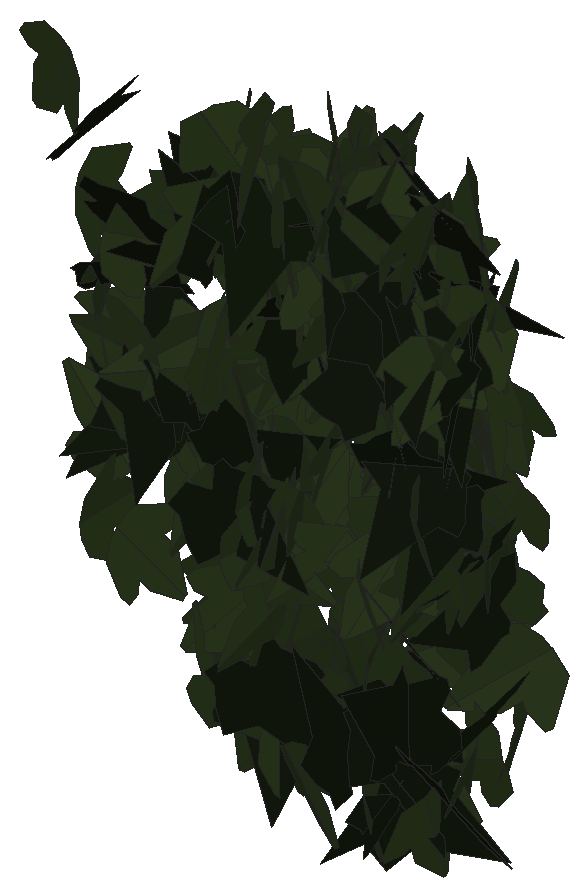
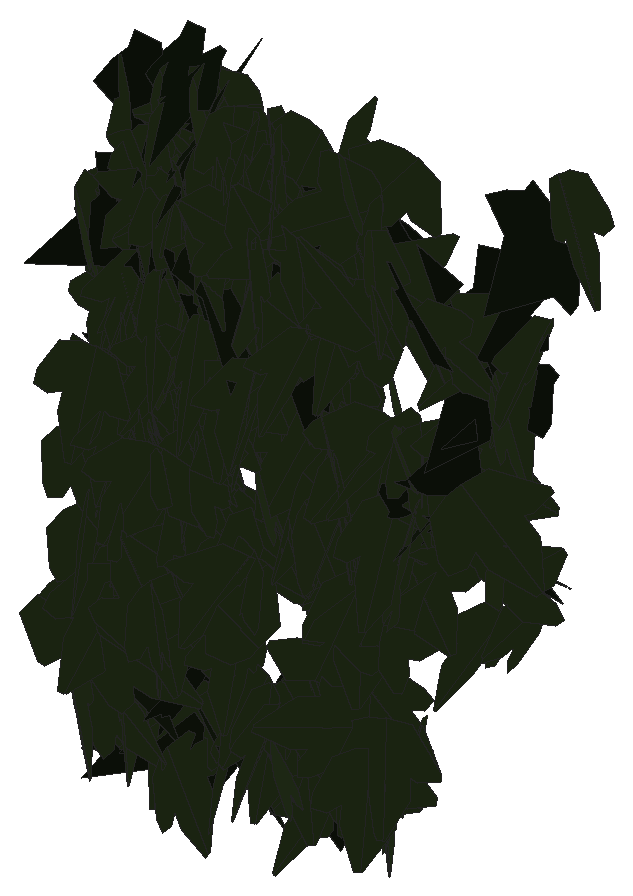
# SketchUp Ruby script. Lengths in inches.
U = 1.inch
M = Sketchup.active_model
def pt(a) = Geom::Point3d.new(a.map { |v| v * U })
def face(e, loops, mat)
  f = e.add_face(loops[0].map { |a| pt(a) })
  loops[1..].each { |l| e.add_face(l.map { |a| pt(a) }).erase! }
  f.material = f.back_material = mat if mat
  f
end
# faces: each face lists its corners as indices into pts; further lists are holes
def faces(e, pts, list, mat = nil) = list.each { |f| face(e, (f[0].is_a?(Array) ? f : [f]).map { |l| l.map { |i| pts[i] } }, mat) }
# xy, xz, yz: faces in a plane at the given z, y or x. An outline is a flat list of corners, or four numbers for a rectangle; further outlines are holes
def ring(l) = l.size == 4 ? [[l[0], l[1]], [l[2], l[1]], [l[2], l[3]], [l[0], l[3]]] : l.each_slice(2).to_a
def flat(e, list, mat, &to3) = list.each { |f| face(e, (f[0].is_a?(Array) ? f : [f]).map { |l| ring(l).map { |u, v| to3.(u, v) } }, mat) }
def xy(e, z, list, mat = nil) = flat(e, list, mat) { |x, y| [x, y, z] }
def xz(e, y, list, mat = nil) = flat(e, list, mat) { |x, z| [x, y, z] }
def yz(e, x, list, mat = nil) = flat(e, list, mat) { |y, z| [x, y, z] }
def lines(e, pts, list) = list.each { |a, b| e.add_line(pt(pts[a]), pt(pts[b])) }
# prism: a flat outline (further loops are holes) pulled along v
def prism(e, loops, v, mat = nil)
  f = face(e, loops, mat); d = Geom::Vector3d.new(v.map { |x| x * U })
  f.pushpull(f.normal.samedirection?(d) ? d.length : -d.length)
end
def box(e, o, s, mat = nil) = prism(e, [[o, [o[0] + s[0], o[1], o[2]], [o[0] + s[0], o[1] + s[1], o[2]], [o[0], o[1] + s[1], o[2]]]], [0, 0, s[2]], mat)
def at(x, y, z, deg = 0) = Geom::Transformation.translation(pt([x, y, z])) * Geom::Transformation.rotation(ORIGIN, Z_AXIS, deg.degrees)
def axes(o, x, y, z) = Geom::Transformation.new([*x, 0, *y, 0, *z, 0, *pt(o).to_a, 1])
def part(name) = M.definitions.add(name)
# library, detail: a bought-in or finely detailed component or shape, given as its bounding box
def library(name, o, s) = part(name).tap { |d| box(d.entities, o, s) }
def detail(e, o, s) = box(e.add_group.entities, o, s)
def put(e, d, t, mat = nil) = e.add_instance(d, t).tap { |i| i.material = mat if mat }
def group(e, t, mat = nil) = e.add_group.tap { |g| g.transformation = t; g.material = mat if mat }.entities
root = M.entities
M.materials.add("efeu1").color = [18, 25, 13]
M.materials.add("efeu2").color = [43, 57, 29]
c1 = part("ivyleaf_10")
p = [[0,0.5,-0.03],[-0.0625,2.02,-0.43],[-0.19,2.01,-0.46],[-0.54,1.05,-0.29],[-0.52,0.625,-0.18],[-0.83,0.76,-0.28],
  [-1.16,0.64,-0.33],[-1.15,0.33,-0.24],[-0.77,-0.39,0.02],[-0.3,-0.51,0.16],[0.04,-0.48,0.23],[-0.02,2.01,-0.4375],
  [-0.06,2.01,-0.43],[0.04,-0.49,0.23],[0.67,-0.49,0.14],[1.38,0.36,-0.2],[1.375,0.51,-0.24],[0.81,0.65,-0.19],
  [0.62,0.59,-0.15],[0.6,1.09,-0.28],[0.5,1.23,-0.31]]
faces(c1.entities,p,[[0,1,2,3,4,5,6,7,8,9,10],[11,12,0,13,14,15,16,17,18,19,20]],"efeu2")
c2 = part("ivyleaf_9")
p = [[1.54,2.16,1.25],[1.36,2.04,1.19],[-0.21,0.99,0.68],[-0.71,1.11,0.82],[-0.85,0.86,0.67],[-0.8,0.17,0.21],
  [-0.9,-0.01,0.1],[-0.67,-0.16,-0.02],[-0.08,-0.08,-0.05],[-0.03,-0.6,-0.4],[0.65,-0.88,-0.66],[0.83,-0.6,-0.49],
  [1.29,-0.42,-0.43],[1.8125,-0.07,-0.26],[1.21,0.44,0.15]]
faces(c2.entities,p,[[0,1,2,3,4,5,6,7,8,9,10,11,12,13,14]],"efeu1")
put(root,c1,axes([5.2,224.04,209.42],[-0.00212,0.02101,0.45187],[-0.16346,0.40731,-0.02119],[-0.44044,-0.15126,0.00569]))
put(root,c2,axes([8.625,224.64,207.9375],[-0.00203,0.05746,0.44843],[-0.23937,-0.37115,0.05043],[0.40424,-0.21948,0.03212]))
put(root,c1,axes([8.18,224.63,208.41],[0.10122,-0.25477,-0.3535],[0.12428,-0.31983,0.28231],[-0.44161,-0.14841,-0.00157]))
put(root,c2,axes([6.96,224.58,213.28],[-0.3714,-0.21956,-0.1569],[0.16606,0.03758,-0.42139],[0.23495,-0.37364,0.04981]))
put(root,c2,axes([8.03,224.45,207.47],[-0.04967,-0.3948,0.18383],[0.04582,0.17278,0.41283],[-0.46492,0.0592,0.02105]))
put(root,c2,axes([8.65,224.39,207.33],[-0.36217,0.27392,-0.04338],[0.03543,-0.02578,-0.45031],[-0.29714,-0.33694,-0.00081]))
put(root,c1,axes([6.83,224.73,208.63],[-0.0006,-0.09982,0.44033],[0.12411,-0.40838,-0.09998],[0.45311,0.11172,0.02797]))
put(root,c1,axes([9.125,224.5,212.34],[0.33338,0.25113,-0.18274],[-0.14436,-0.11411,-0.41383],[-0.29788,0.33636,-0.00396]))
put(root,c2,axes([8.61,224.53,212.71],[-0.21473,-0.29356,-0.2621],[0.19877,0.17748,-0.36601],[0.36755,-0.26748,0.04481]))
put(root,c1,axes([5.54,224.2,209.1875],[0.02158,0.3425,0.27813],[0.0277,0.26632,-0.35671],[-0.46849,0.03152,-0.00828]))
put(root,c1,axes([7.42,224.48,207.21],[-0.31943,0.21184,-0.24801],[0.21615,-0.12999,-0.37824],[-0.26825,-0.357,-0.00945]))
put(root,c2,axes([9,224.62,211.02],[-0.44478,-0.12881,-0.05722],[0.05701,0.01553,-0.44877],[0.14012,-0.4152,0.00096]))
put(root,c2,axes([5.45,224.73,210.68],[-0.06726,-0.41548,0.11732],[-0.00699,-0.11306,-0.4368],[0.46491,-0.06181,0.0104]))
put(root,c2,axes([6.42,224.41,209.95],[-0.03075,-0.08309,-0.44308],[0.34115,0.28887,-0.08054],[0.32153,-0.31444,0.04308]))
put(root,c2,axes([9.26,224.625,210.84],[-0.4243,-0.04481,-0.18856],[0.19735,-0.00503,-0.41051],[0.04165,-0.43266,0.02431]))
put(root,c1,axes([7.2,224.33,209.67],[0.19213,-0.3133,0.25351],[-0.13025,0.21183,0.3747],[-0.40845,-0.21493,-0.00024]))
put(root,c2,axes([8.36,224.52,211.6875],[-0.29043,-0.32348,0.1152],[0.08307,0.08008,0.43741],[-0.35981,0.27959,0.008]))
put(root,c2,axes([4.99,224.41,212.74],[0.41192,-0.06876,0.20544],[0.21519,-0.00554,-0.40211],[0.06873,0.42949,0.0277]))
put(root,c1,axes([8.57,224.42,211.875],[-0.27605,0.34528,0.07114],[-0.05347,0.04843,-0.44663],[-0.37637,-0.26012,0.01127]))
put(root,c1,axes([8.91,224.66,213.81],[0.06813,-0.41929,0.10105],[0.03005,-0.09403,-0.44076],[0.46386,0.06767,0.01371]))
put(root,c1,axes([4.42,224.42,214.15],[0.37791,-0.15784,-0.28682],[-0.19638,0.2412,-0.39148],[0.26194,0.40855,0.12031]))
put(root,c1,axes([9.07,224.31,210.6],[-0.21616,0.22463,0.32675],[-0.23093,0.23023,-0.31286],[-0.34736,-0.29285,0.00466]))
put(root,c1,axes([6.65,224.53,211.17],[-0.27348,0.34702,-0.07117],[0.04419,-0.05486,-0.44677],[-0.37943,-0.2565,-0.00074]))
put(root,c1,axes([9,224.5,207.23],[-0.06491,-0.40687,-0.14734],[0.08934,0.12949,-0.42324],[0.45664,-0.08317,0.06186]))
put(root,c2,axes([6.4,224.38,212.75],[-0.04797,0.10555,0.43644],[-0.2722,0.33661,-0.11579],[-0.37989,-0.25452,0.02785]))
put(root,c1,axes([8.98,224.54,210.05],[-0.41664,0.00882,0.20883],[-0.21705,-0.02308,-0.40051],[0.00307,-0.4343,0.02552]))
put(root,c1,axes([6.11,224.89,212.86],[-0.08756,-0.30933,0.38295],[-0.07097,-0.37696,-0.32072],[0.48713,-0.11052,0.02211]))
put(root,c1,axes([5.1,224.55,209.96],[0.34077,0.14902,0.33417],[-0.33927,-0.04231,0.36484],[0.13702,-0.4754,0.07228]))
put(root,c2,axes([6.86,224.53,208.05],[-0.11147,-0.11457,-0.42302],[0.27588,0.31663,-0.16017],[0.36356,-0.2754,-0.00816]))
put(root,c1,axes([6.62,224.88,213.97],[0.15051,-0.30432,0.36707],[0.22118,-0.29644,-0.33645],[0.4224,0.26366,0.04539]))
put(root,c1,axes([6.81,224.63,209.32],[-0.14118,-0.00993,-0.43137],[0.43765,-0.09638,-0.13042],[-0.09616,-0.42407,0.03974]))
put(root,c2,axes([8.59,224.92,212.67],[-0.07873,-0.39699,0.16868],[-0.02446,-0.16073,-0.41973],[0.46251,-0.07608,0.00651]))
put(root,c1,axes([6.9,224.91,209.53],[0.0196,0.15172,-0.42357],[-0.07247,-0.40177,-0.15876],[-0.46376,0.06919,0.00691]))
put(root,c1,axes([5.33,224.52,211.09],[0.03073,-0.02803,-0.49827],[-0.45328,0.20729,-0.03962],[0.20879,0.45414,-0.01267]))
put(root,c1,axes([7.15,224.62,211.98],[-0.25446,-0.36382,-0.03815],[0.02817,0.02681,-0.45072],[0.39392,-0.23694,0.00759]))
put(root,c1,axes([7.36,224.61,213.74],[-0.42398,0.15176,-0.11432],[0.10621,-0.05035,-0.43756],[-0.17227,-0.40455,0.01157]))
put(root,c2,axes([5.38,224.81,210.63],[-0.46047,-0.08538,0.01283],[-0.01184,-0.00804,-0.45218],[0.09241,-0.42646,0.00596]))
put(root,c1,axes([8.98,224.58,212.38],[-0.44344,0.1425,0.01902],[-0.01907,0.00491,-0.452],[-0.15398,-0.41097,0.0012]))
put(root,c2,axes([4.77,224.28,213.54],[0.15081,0.29111,0.30317],[0.05059,0.29458,-0.32929],[-0.44205,0.13303,0.06574]))
put(root,c1,axes([7.69,224.85,209.49],[-0.16495,-0.19077,0.37426],[-0.23325,-0.28793,-0.25406],[0.37296,-0.26445,0.00663]))
put(root,c1,axes([7,224.6,210.08],[-0.49258,-0.02674,0.08155],[-0.08138,-0.00531,-0.4933],[0.02725,-0.49926,0.00088]))
put(root,c2,axes([8.68,224.44,207.3],[0.02609,-0.03815,-0.44996],[0.14664,0.41226,-0.02992],[0.44556,-0.13345,0.0362]))
put(root,c2,axes([5.13,224.37,212.15],[0.33379,0.28979,0.10256],[0.05012,0.09417,-0.43903],[-0.32678,0.31045,0.03743]))
put(root,c1,axes([8.38,224.44,207.17],[-0.18335,0.31626,0.25556],[-0.15375,0.20181,-0.37241],[-0.40429,-0.22018,0.02573]))
put(root,c1,axes([7.74,224.59,213.72],[0.19435,-0.41858,-0.19242],[-0.05741,0.1852,-0.46087],[0.45709,0.20123,0.02393]))
put(root,c1,axes([8.28,224.51,213.81],[-0.06856,-0.05507,-0.44388],[0.43369,0.14754,-0.08191],[0.16711,-0.40549,0.03048]))
put(root,c1,axes([5.75,224.98,210.94],[-0.01762,0.06632,0.49527],[-0.18417,-0.46155,0.05526],[0.46451,-0.18048,0.0407]))
put(root,c1,axes([8.36,224.75,209.7],[0.38435,0.16569,-0.19491],[-0.18173,-0.08258,-0.40824],[-0.1999,0.39364,-0.00361]))
put(root,c2,axes([8.43,224.7,207.97],[0.13367,-0.43867,-0.19924],[-0.04143,0.19554,-0.45831],[0.48002,0.13903,0.01593]))
put(root,c2,axes([8.47,224.63,210.76],[0.16775,-0.07991,0.41432],[0.42497,-0.07677,-0.17557],[0.10943,0.42065,0.04667]))
put(root,c1,axes([6.89,224.52,212.78],[-0.327,0.1813,0.2645],[-0.24508,0.11569,-0.36673],[-0.23177,-0.37812,0.01461]))
put(root,c2,axes([9.23,224.46,212.06],[-0.29735,0.33575,0.02738],[0.01248,-0.02457,0.45152],[0.36351,0.27548,0.0069]))
put(root,c1,axes([6.23,224.67,213.9],[-0.35741,-0.11571,-0.26783],[0.29682,-0.04122,-0.34804],[0.06978,-0.4173,0.10864]))
put(root,c1,axes([7.09,224.7,213.35],[-0.07337,0.41948,-0.09669],[0.01735,-0.09158,-0.44195],[-0.46371,-0.0698,-0.00123]))
put(root,c1,axes([6.97,224.73,207.53],[-0.36305,-0.16965,0.22652],[-0.21118,-0.09597,-0.3916],[0.2105,-0.38889,-0.00218]))
put(root,c2,axes([8.97,224.7,208.27],[-0.14213,0.01117,-0.43104],[-0.39914,-0.20027,0.11643],[-0.20298,0.386,0.07288]))
put(root,c2,axes([6.46,224.65,210.15],[0.01791,0.00244,0.45206],[0.44631,-0.135,-0.01561],[0.1456,0.41351,-0.00777]))
put(root,c2,axes([8.22,224.66,209.26],[0.43399,-0.16623,-0.01114],[-0.0101,0.00539,-0.45226],[0.17962,0.40195,0.00146]))
put(root,c2,axes([5.53,224.9,210.54],[-0.46135,0.00633,0.08515],[-0.08726,-0.10996,-0.42956],[0.01586,-0.42082,0.11353]))
put(root,c2,axes([8.68,224.72,207.46],[0.40917,-0.18,0.11988],[0.11632,-0.04185,-0.43615],[0.1994,0.39379,0.00844]))
put(root,c1,axes([6.91,224.7,212.68],[-0.46596,-0.00698,-0.05724],[0.05981,-0.02834,-0.44775],[0.00359,-0.43402,0.03016]))
put(root,c2,axes([8.53,225.09,213.37],[0.2317,-0.4172,-0.14919],[0.06983,-0.13187,0.47721],[-0.43754,-0.24198,-0.00285]))
put(root,c1,axes([4.84,224.85,212.12],[0.14378,-0.47608,0.05171],[0.02083,-0.04772,-0.49728],[0.47843,0.14516,0.00611]))
put(root,c2,axes([9.07,224.61,213.89],[0.42077,0.05332,-0.19343],[-0.1997,-0.02051,-0.40894],[-0.06152,0.43123,0.00446]))
put(root,c1,axes([6.72,224.42,209.39],[0.01931,-0.04767,0.44929],[-0.04052,0.43059,0.05103],[-0.46765,-0.03927,0.01413]))
put(root,c1,axes([8.57,224.74,208.58],[-0.37115,-0.03785,0.27455],[-0.28083,-0.04808,-0.35921],[0.06397,-0.43067,0.01597]))
put(root,c1,axes([6.83,224.4375,209.95],[-0.03174,0.02521,0.4506],[-0.21761,0.38384,-0.03744],[-0.41515,-0.20312,-0.01482]))
put(root,c2,axes([9.01,224.88,212.24],[-0.25835,-0.09434,-0.36489],[0.37452,0.06604,-0.26435],[0.11707,-0.41948,0.04045]))
put(root,c2,axes([7.22,224.58,212.11],[0.17541,-0.17371,-0.37881],[-0.16634,0.33623,-0.23819],[0.40283,0.21447,0.0666]))
put(root,c1,axes([6.4375,224.91,213.06],[-0.19956,0.07607,0.40184],[0.39351,-0.12892,0.20761],[0.16137,0.40843,-0.00932]))
put(root,c1,axes([5.27,224.42,212.46],[0.03353,0.19812,0.45785],[0.0002,0.45887,-0.19858],[-0.49887,0.0135,0.03069]))
put(root,c1,axes([5.09,224.64,210.27],[-0.21597,0.39315,-0.22089],[-0.14918,0.16883,0.44636],[0.42556,0.2587,0.04438]))
put(root,c1,axes([5.89,224.93,211.0625],[0.26574,-0.3409,-0.25134],[0.16122,-0.19296,0.43217],[-0.39165,-0.31073,0.00737]))
put(root,c1,axes([7.24,225,211.85],[0.10835,0.34406,-0.34625],[-0.19149,-0.29628,-0.35433],[-0.44899,0.20938,0.06756]))
put(root,c1,axes([7.19,224.74,209.75],[0.44549,-0.02798,-0.22529],[0.22617,0.01173,0.44577],[-0.01966,-0.49908,0.0231]))
put(root,c1,axes([8.1875,225.02,213.4],[0.14785,-0.30566,0.28869],[0.2035,-0.21397,-0.34168],[0.39679,0.22363,0.06767]))
put(root,c1,axes([7,224.79,212.31],[0.38955,-0.20629,-0.13389],[-0.08711,0.11577,-0.42794],[0.24775,0.36506,0.06006]))
put(root,c1,axes([8.3,224.93,214.04],[0.17044,-0.46418,0.0741],[0.02779,-0.06873,-0.49447],[0.46923,0.17268,0.00237]))
put(root,c1,axes([8.17,224.61,209.42],[-0.24585,0.27669,0.25654],[-0.16738,0.19192,-0.37262],[-0.36366,-0.27539,-0.00193]))
put(root,c1,axes([8.6,224.76,207.6],[-0.33002,-0.03883,-0.31944],[0.33215,0.01154,-0.31972],[0.03844,-0.43311,0.02012]))
put(root,c1,axes([6.37,224.85,208.54],[0.37569,-0.0578,-0.26489],[-0.27284,0.0332,-0.36667],[0.07159,0.42986,-0.0073]))
put(root,c1,axes([8.71,225.19,209.61],[0.06423,-0.19278,0.45685],[0.12341,-0.43996,-0.203],[0.48025,0.13884,-0.00894]))
put(root,c2,axes([6.86,224.95,207.61],[-0.31949,-0.24683,-0.21004],[0.16409,0.13313,-0.40066],[0.30285,-0.33253,-0.0045]))
put(root,c1,axes([6.55,224.6,212.49],[-0.06999,-0.22087,0.38387],[0.10197,0.35687,0.23933],[-0.45323,0.1144,-0.00543]))
put(root,c1,axes([8.53,224.59,210.75],[0.06364,-0.06369,0.44331],[-0.34178,0.28567,0.08989],[-0.31599,-0.32181,-0.00794]))
put(root,c1,axes([9.28,224.96,212.66],[0.30382,0.12049,-0.37838],[-0.36131,-0.11381,-0.32635],[-0.16477,0.47173,0.01792]))
put(root,c2,axes([8,224.84,213.48],[0.12503,-0.36763,-0.20975],[-0.00294,0.20856,-0.397],[0.45285,0.10285,0.05533]))
put(root,c1,axes([9.14,224.96,212.49],[0.1133,-0.41547,0.07788],[0.02341,-0.07176,-0.44563],[0.45533,0.10707,0.00353]))
put(root,c1,axes([7.45,224.78,213.16],[-0.36927,0.26863,-0.01304],[0.01235,-0.00573,-0.4522],[-0.29017,-0.3421,-0.00266]))
put(root,c1,axes([7.49,224.82,212.5],[0.29174,0.33816,0.04536],[0.03742,0.02814,-0.45001],[-0.36633,0.27218,-0.00984]))
put(root,c1,axes([7.69,225.13,211.91],[-0.20093,-0.33012,0.31726],[-0.00932,-0.34344,-0.36326],[0.45776,-0.15189,0.13186]))
put(root,c1,axes([8.77,224.89,213.41],[0.44915,-0.10978,0.06752],[0.08206,0.03542,-0.44392],[0.11063,0.41943,0.05516]))
put(root,c2,axes([9,225.06,212.42],[-0.24416,0.03874,-0.43461],[0.42235,-0.10408,-0.24655],[-0.10957,-0.48751,0.0181]))
put(root,c1,axes([8.71,224.88,213.625],[-0.0254,-0.43114,-0.0549],[-0.00103,0.05291,-0.44904],[0.46911,-0.02322,-0.00396]))
put(root,c1,axes([7.76,224.77,212.33],[-0.12216,-0.44162,-0.20013],[0.0466,0.19473,-0.45816],[0.4826,-0.13059,-0.00642]))
put(root,c1,axes([7.52,224.79,212.9],[-0.29779,0.0688,0.34251],[-0.35358,0.04327,-0.29446],[-0.08374,-0.42734,0.02533]))
put(root,c2,axes([5.54,224.92,210.8],[0.26318,-0.35282,-0.07614],[-0.00624,0.08455,-0.44373],[0.38911,0.23999,0.04439]))
put(root,c1,axes([6.83,224.9,210.53],[-0.35443,0.17208,-0.23696],[0.22006,-0.10202,-0.38536],[-0.21602,-0.38627,-0.00378]))
put(root,c2,axes([8.55,224.71,214.3],[0.39474,-0.00034,-0.24531],[-0.24622,0.1111,-0.36756],[0.06536,0.42057,0.0969]))
put(root,c2,axes([6.83,225.0625,211.98],[0.08714,-0.00464,-0.44452],[0.4606,-0.02844,0.08405],[-0.03111,-0.43404,-0.00076]))
put(root,c1,axes([4.67,224.66,212.67],[-0.12175,0.407,0.26368],[-0.07342,0.25326,-0.42482],[-0.47936,-0.14216,-0.0019]))
put(root,c1,axes([6.09,224.875,207.38],[-0.19525,0.45979,-0.02157],[-0.02216,0.01402,0.49931],[0.45977,0.19594,0.0149]))
put(root,c1,axes([8.58,225.1,209.52],[-0.02268,-0.40103,0.17389],[-0.01151,-0.16687,-0.41764],[0.46911,-0.02348,-0.00184]))
put(root,c1,axes([7.23,225.06,211.16],[-0.36245,-0.17766,0.22069],[-0.1446,-0.18769,-0.38363],[0.2616,-0.3499,0.09373]))
put(root,c1,axes([6.11,224.99,207.8],[-0.32105,0.29762,-0.24156],[0.17558,-0.16591,-0.43777],[-0.34073,-0.36592,0.00202]))
put(root,c2,axes([7.01,224.71,212.89],[0.38981,0.24014,0.03726],[0.02339,0.03208,-0.45061],[-0.26118,0.36129,0.01525]))
put(root,c1,axes([6.84,224.68,212.4],[-0.01586,0.30717,0.31997],[-0.05421,0.30458,-0.31875],[-0.46639,-0.04585,0.02617]))
put(root,c1,axes([5.7,225.31,209.59],[-0.05433,-0.24121,0.43459],[0.16513,-0.4211,-0.21308],[0.46881,0.12038,0.12542]))
put(root,c1,axes([9.04,224.91,210.79],[-0.46246,0.05487,-0.05557],[0.05657,-0.01161,-0.44895],[-0.06035,-0.43137,0.00501]))
put(root,c1,axes([7.31,224.67,210.22],[0.05179,-0.2562,-0.42624],[-0.02712,0.42645,-0.25962],[0.49657,0.05001,0.03028]))
put(root,c1,axes([8.48,224.92,211.62],[0.17781,-0.05389,-0.41498],[0.43435,0.00123,0.17241],[-0.02096,-0.43165,0.0523]))
put(root,c1,axes([7.7,224.98,213.29],[-0.35546,-0.05734,-0.28973],[0.30716,-0.07124,-0.3342],[-0.00353,-0.42528,0.09505]))
put(root,c2,axes([5.66,224.95,210.78],[-0.33509,-0.27565,0.13549],[0.11887,0.07208,0.43121],[-0.30707,0.32871,0.01906]))
put(root,c1,axes([6.72,225.27,210.72],[-0.06006,-0.36381,0.33769],[0.16152,-0.33597,-0.33322],[0.46937,0.06906,0.15788]))
put(root,c1,axes([5.69,224.99,211.35],[-0.12749,-0.41841,-0.01545],[0.00685,0.01364,-0.45213],[0.45212,-0.11819,0.00249]))
put(root,c1,axes([7.91,224.99,212.58],[-0.28255,-0.34383,-0.05266],[0.09561,-0.00464,-0.44291],[0.36296,-0.26643,0.07568]))
put(root,c1,axes([8.46,225.0625,212.88],[-0.06493,-0.42628,0.0649],[-0.01932,-0.06048,-0.44762],[0.46489,-0.06205,-0.00953]))
put(root,c2,axes([9.51,224.97,209.53],[-0.3996,0.20329,0.10907],[-0.0945,0.05848,-0.43896],[-0.22826,-0.3801,-0.0092]))
put(root,c1,axes([8.44,224.92,213.45],[-0.46633,0.051,-0.01419],[0.01613,0.01022,-0.45201],[-0.05469,-0.43188,-0.01237]))
put(root,c2,axes([7.16,224.81,212.3],[0.07416,0.42628,-0.05497],[-0.01083,-0.05192,-0.44904],[-0.46378,0.06937,0.00169]))
put(root,c1,axes([7.65,225.25,212.58],[-0.10271,0.2291,0.37164],[0.04114,-0.36012,0.25066],[0.45658,0.08399,0.06102]))
put(root,c1,axes([7.35,225.17,210.59],[0.18779,-0.43739,0.15307],[0.06579,-0.13832,-0.47596],[0.4587,0.1989,0.0056]))
put(root,c1,axes([4.92,225.19,211.08],[-0.2999,-0.25897,0.30496],[-0.18471,-0.24845,-0.39263],[0.35488,-0.34815,0.05335]))
put(root,c1,axes([5.63,224.97,212.54],[0.17303,-0.06332,-0.41541],[-0.40333,0.14172,-0.17915],[0.16763,0.40636,-0.00225]))
put(root,c1,axes([5.75,225.05,210.06],[0.33637,0.27066,-0.14323],[-0.1697,-0.02519,-0.42104],[-0.28066,0.33961,0.08292]))
put(root,c1,axes([8.63,225,213.43],[-0.43512,-0.14722,-0.07521],[0.08535,-0.00615,-0.44483],[0.15523,-0.40928,0.03374]))
put(root,c1,axes([6.24,225.29,210.3],[0.07879,-0.1693,0.46382],[0.39193,-0.26423,-0.16303],[0.30031,0.38926,0.09107]))
put(root,c1,axes([6.85,225.04,211.77],[-0.26762,-0.33694,-0.12433],[0.20746,-0.0028,-0.40589],[0.32565,-0.27512,0.1564]))
put(root,c1,axes([8.49,225.04,212.96],[-0.28227,-0.34755,-0.01183],[0.01401,0.00447,-0.45217],[0.37529,-0.26157,0.00799]))
put(root,c1,axes([6.96,224.76,207.22],[-0.00424,0.29694,0.33058],[-0.01819,0.31753,-0.30871],[-0.46943,-0.01499,0.00898]))
put(root,c2,axes([8.58,225.12,213.08],[0.09123,-0.38404,0.19345],[-0.01801,0.1865,0.40834],[-0.4605,-0.08338,0.02236]))
put(root,c1,axes([8.42,225.17,207.11],[-0.00042,-0.4214,0.11223],[0.00308,-0.10791,-0.43825],[0.46979,0.00033,0.00297]))
put(root,c1,axes([9.28,225.09,209.8],[-0.01751,-0.43469,0.00177],[-0.00025,-0.0017,-0.4524],[0.46947,-0.01622,-0.00017]))
put(root,c2,axes([9.43,225.03,208.26],[-0.27593,0.34401,-0.07787],[-0.01377,-0.10149,-0.43972],[-0.37998,-0.24613,0.07248]))
put(root,c1,axes([8.04,225.24,211.83],[0.16037,0.15087,-0.39522],[-0.33886,-0.21719,-0.21718],[-0.28314,0.34538,0.03606]))
put(root,c2,axes([9.24,224.79,209.88],[-0.01079,0.38935,0.20149],[-0.12605,0.18428,-0.39141],[-0.45245,-0.06063,0.10424]))
put(root,c1,axes([7.73,225.27,212.79],[-0.26677,-0.15304,0.33666],[-0.21024,-0.27268,-0.28855],[0.32457,-0.30241,0.0898]))
put(root,c1,axes([6.72,225.11,209.8],[-0.14443,0.40778,0.07394],[0.01856,-0.06918,0.44628],[0.44666,0.13473,0.00536]))
put(root,c1,axes([8.82,225.21,211.13],[0.29194,-0.32434,0.10888],[0.0807,-0.07397,-0.43898],[0.35913,0.28028,0.01014]))
put(root,c1,axes([6.66,225.18,211.375],[0.23507,-0.37502,0.03615],[0.03464,-0.02155,-0.45061],[0.40528,0.21936,0.01754]))
put(root,c1,axes([8.89,224.77,212.55],[0.10951,0.0869,-0.43055],[0.05948,0.41939,0.10559],[0.45297,-0.07608,0.09023]))
put(root,c1,axes([7.04,225.1,207.82],[-0.44028,-0.10567,0.11331],[-0.11351,-0.02873,-0.43798],[0.11825,-0.42099,0.00145]))
put(root,c1,axes([6.83,225.17,208.61],[0.29713,-0.33623,-0.02296],[-0.01482,0.01729,-0.45182],[0.36361,0.27546,0.00035]))
put(root,c2,axes([8.06,225.06,212.375],[-0.28264,0.34646,-0.02758],[0.01532,-0.02253,-0.45155],[-0.37496,-0.26208,0.00235]))
put(root,c1,axes([9.15,225.02,207.6875],[0.11178,-0.35891,-0.23184],[-0.07048,0.21318,-0.38846],[0.45083,0.12231,-0.00325]))
put(root,c1,axes([9.03,225.13,212.8],[-0.41416,0.19104,-0.20486],[0.17704,-0.10487,-0.4557],[-0.21709,-0.45001,0.01922]))
put(root,c1,axes([8.81,225.02,212.47],[-0.38343,0.21927,0.12781],[-0.12258,0.04992,-0.43363],[-0.24222,-0.37236,0.01713]))
put(root,c1,axes([8.86,225.15,211.5],[-0.41843,-0.04939,0.19918],[-0.19529,-0.0822,-0.40248],[0.08655,-0.4243,0.05479]))
put(root,c1,axes([8.67,225.01,212.72],[-0.27168,0.32573,0.14651],[-0.1298,0.08428,-0.42586],[-0.36063,-0.27572,0.0429]))
put(root,c1,axes([6.3,225.09,212.5],[0.32819,0.01225,0.37701],[0.35931,0.14196,-0.3174],[-0.11482,0.47927,0.08438]))
put(root,c1,axes([8.07,225.15,211.71],[-0.00819,0.42855,-0.07719],[-0.01694,-0.07446,-0.44543],[-0.46942,-0.00479,0.01742]))
put(root,c1,axes([6.6,224.97,212.51],[-0.07583,-0.40524,-0.2829],[0.0399,0.28025,-0.41215],[0.4926,-0.08508,-0.01016]))
put(root,c1,axes([8.83,225.35,213.75],[0.20893,-0.13435,0.43393],[0.40128,-0.16925,-0.24562],[0.21289,0.45089,0.0371]))
put(root,c1,axes([6.1875,224.99,207.83],[0.15562,-0.31923,-0.35196],[-0.16313,0.31195,-0.35507],[0.44628,0.22535,-0.00706]))
put(root,c1,axes([7.55,225.11,213.76],[0.13855,-0.4488,-0.1714],[-0.02394,0.17172,-0.46898],[0.47982,0.13816,0.02609]))
put(root,c1,axes([7.32,225.22,210.13],[0.28695,0.30446,-0.1675],[-0.17811,-0.06613,-0.41294],[-0.32657,0.30358,0.07803]))
put(root,c1,axes([7.8125,225.11,213.97],[-0.11965,-0.40129,-0.1312],[0.02685,0.12398,-0.43287],[0.45351,-0.11321,-0.00899]))
put(root,c1,axes([7.54,225.16,208.22],[-0.41095,0.17796,-0.11751],[0.1076,-0.05365,-0.43683],[-0.20063,-0.39329,0.00642]))
put(root,c1,axes([9.12,225.08,211.88],[-0.19767,0.39072,0.05757],[-0.01652,0.05395,-0.44863],[-0.42587,-0.18345,-0.00932]))
put(root,c1,axes([7.11,225.36,212.45],[-0.18903,-0.20641,0.35419],[-0.24345,-0.25532,-0.28142],[0.35455,-0.28536,-0.0044]))
put(root,c1,axes([6.08,225.375,208.02],[0.03055,0.30751,-0.31863],[-0.16893,-0.27918,-0.30644],[-0.43731,0.12933,0.09611]))
put(root,c2,axes([7.55,225.08,211.76],[0.26961,0.35459,-0.03561],[0.00507,0.03854,0.45059],[0.3847,-0.24901,0.01902]))
put(root,c1,axes([7.59,225.15,213.12],[-0.46889,-0.0137,0.02427],[-0.02501,-0.0062,-0.45171],[0.01513,-0.43474,0.00568]))
put(root,c1,axes([9.11,225.11,211.65],[-0.24938,0.36709,0.03527],[-0.02276,0.02681,-0.45101],[-0.39749,-0.23184,0.0037]))
put(root,c1,axes([9.16,225.31,211.72],[-0.39143,0.16376,-0.18325],[0.09378,-0.2081,-0.38688],[-0.24228,-0.34511,0.14632]))
put(root,c1,axes([7,225.41,207.89],[0.16711,-0.34268,0.2275],[0.11071,-0.19361,-0.39084],[0.42489,0.18523,0.01236]))
put(root,c1,axes([5.96,224.91,211.25],[-0.00786,-0.21957,-0.44914],[0.19075,0.4139,-0.20568],[0.46212,-0.17458,0.07726]))
put(root,c1,axes([9.375,224.9375,210.08],[0.127,-0.08086,-0.42736],[-0.11325,0.40754,-0.11461],[0.4379,0.12884,0.0943]))
put(root,c1,axes([8.91,225.26,212],[0.23724,-0.3718,-0.05442],[-0.03106,0.04378,-0.44911],[0.40431,0.22153,-0.00257]))
put(root,c2,axes([8.74,225.03,212.76],[0.41927,0.05152,0.19694],[0.19308,0.08028,-0.40389],[-0.08742,0.42441,0.0525]))
put(root,c1,axes([7.08,225.2,208.29],[-0.2865,-0.01515,0.35819],[-0.37149,-0.01757,-0.27634],[0.02502,-0.43438,-0.00131]))
put(root,c1,axes([9.28,225.1875,207.62],[-0.16423,0.03629,0.42217],[-0.44003,-0.00301,-0.15845],[-0.01069,-0.43347,0.03644]))
put(root,c1,axes([7.85,225.39,213.77],[-0.03163,-0.40951,0.14951],[0.04051,-0.14594,-0.42439],[0.46698,-0.01508,0.04695]))
put(root,c1,axes([7.37,224.96,211.09],[0.1773,0.10748,0.40376],[0.14235,0.38182,-0.16791],[-0.41111,0.17857,0.11599]))
put(root,c1,axes([7.55,225.04,213.67],[-0.17242,0.34429,0.22112],[-0.118,0.1834,-0.39418],[-0.42079,-0.1925,0.01993]))
put(root,c1,axes([7.87,225.57,212.81],[-0.02576,-0.032,-0.45049],[0.0303,-0.43302,0.03167],[-0.46811,-0.02627,0.02684]))
put(root,c1,axes([6.6,225.4,210.4],[0.04207,-0.48341,0.12059],[0.004,-0.12069,-0.4852],[0.49821,0.04179,-0.00628]))
put(root,c1,axes([8.35,225.22,213.29],[0.2371,-0.34353,-0.15778],[-0.07712,0.13434,-0.42383],[0.39818,0.23058,0.01186]))
put(root,c1,axes([5.875,225.18,209.9],[-0.25926,0.41759,-0.09168],[-0.04908,0.07744,0.49152],[0.4247,0.26387,0.00084]))
put(root,c1,axes([6.58,224.9,213.48],[0.00865,0.02198,0.49944],[0.12108,0.48455,-0.02342],[-0.48504,0.12135,0.00307]))
put(root,c1,axes([8.9375,225.03,209.73],[0.12689,-0.25466,-0.34582],[0.01799,0.34792,-0.271],[0.45198,0.05765,0.10787]))
put(root,c1,axes([8.86,225.25,209.15],[-0.2765,-0.34955,-0.04019],[0.02886,0.02833,-0.45058],[0.37871,-0.25737,0.005]))
put(root,c1,axes([8.4,225.38,210.56],[0.35503,-0.27147,0.08985],[0.06596,-0.06169,-0.4433],[0.30053,0.33425,-0.00885]))
put(root,c1,axes([7.38,225.31,209.89],[0.15456,-0.03379,-0.42577],[0.42448,-0.11478,0.15274],[-0.12898,-0.41822,-0.00752]))
put(root,c1,axes([6.95,225.21,211.09],[-0.44456,-0.02935,-0.14308],[0.14849,0.00602,-0.42916],[0.03213,-0.43397,0.00372]))
put(root,c1,axes([6.52,225.23,210.92],[0.29341,-0.37558,-0.15115],[-0.05723,0.14632,-0.47467],[0.40079,0.29585,0.04287]))
put(root,c1,axes([6.11,225.16,211.35],[-0.40658,-0.11484,-0.2674],[0.25367,0.08531,-0.42234],[0.14263,-0.4791,-0.01111]))
put(root,c1,axes([7.26,225.17,208.12],[-0.12826,-0.4434,-0.19223],[0.04503,0.18705,-0.4615],[0.48117,-0.13569,-0.00805]))
put(root,c2,axes([5.83,225.04,212.74],[-0.11367,0.18958,0.39219],[-0.19359,0.33179,-0.2255],[-0.41269,-0.20786,-0.00225]))
put(root,c1,axes([7.58,225.18,214],[-0.22598,0.37282,0.08352],[-0.07546,0.05258,-0.44317],[-0.40491,-0.21787,0.03598]))
put(root,c1,axes([8.61,225.13,213.03],[0.23657,0.25858,0.28364],[0.185,0.21228,-0.3524],[-0.36128,0.27802,0.00527]))
put(root,c1,axes([8.43,225.36,211.29],[-0.27101,0.33375,0.12682],[0.0748,-0.10048,0.43423],[0.37639,0.26027,0.00502]))
put(root,c1,axes([8.45,225.41,210.59],[0.30098,-0.32572,0.07687],[0.04503,-0.06159,-0.44574],[0.3579,0.28167,-0.00857]))
put(root,c1,axes([8.45,225.19,210.55],[-0.13331,-0.34596,0.24234],[0.07579,0.22232,0.38194],[-0.44407,0.1418,-0.00756]))
put(root,c1,axes([8.86,225.23,211.34],[-0.43551,0.15692,0.04643],[-0.043,0.02078,-0.44998],[-0.17087,-0.40518,-0.0051]))
put(root,c1,axes([8.16,225.375,210.51],[0.46949,0.01521,-0.00412],[-0.00372,-0.01476,-0.45213],[-0.01656,0.43448,-0.01522]))
put(root,c1,axes([5.87,225.23,210.61],[-0.21056,-0.42033,-0.17025],[0.08903,0.14574,-0.46993],[0.44468,-0.22821,0.01347]))
put(root,c1,axes([6.14,225.32,209.76],[-0.32208,-0.38157,-0.02585],[0.01695,0.01952,-0.49933],[0.38207,-0.32253,0.00036]))
put(root,c1,axes([8.85,225.21,212.22],[0.06383,0.41372,0.12554],[-0.0498,0.12721,-0.42996],[-0.46277,0.04338,0.06358]))
put(root,c1,axes([9.22,225.46,209.51],[-0.33784,-0.19396,0.24112],[-0.17616,-0.17259,-0.37904],[0.27485,-0.34902,0.05344]))
put(root,c1,axes([8.01,225.48,210.72],[-0.26279,-0.31392,0.18449],[-0.10723,-0.1474,-0.41292],[0.37437,-0.26258,0.01124]))
put(root,c1,axes([7.27,225.15,213.91],[0.13349,-0.21386,-0.37239],[-0.1048,0.34847,-0.25129],[0.43808,0.14853,0.05336]))
put(root,c1,axes([9.27,225.47,212.82],[0.2037,-0.38812,0.05709],[0.04632,-0.04012,-0.44826],[0.4208,0.1923,0.02171]))
put(root,c1,axes([9.11,225.43,211.23],[0.45937,-0.08631,-0.03047],[-0.0306,0.0077,-0.45137],[0.09356,0.42628,0.00199]))
put(root,c1,axes([8.41,225.65,209.34],[-0.10475,-0.30516,0.30621],[-0.04116,-0.29454,-0.33054],[0.45612,-0.09666,0.04049]))
put(root,c2,axes([7.8,225.15,212.54],[-0.00292,0.41325,0.14123],[-0.05398,0.13461,-0.42704],[-0.46668,-0.01816,0.04851]))
put(root,c1,axes([8.78,225.38,210.96],[0.25189,-0.3328,-0.16135],[-0.05701,0.1515,-0.42051],[0.39244,0.23562,0.04248]))
put(root,c1,axes([7.57,225.57,211.27],[0.23997,-0.28726,-0.24903],[0.1621,-0.18661,0.37767],[-0.36993,-0.26811,0.00395]))
put(root,c1,axes([6.65,225.5,213.22],[0.48241,-0.00873,0.13115],[0.13095,-0.01124,-0.48242],[0.01137,0.4998,-0.00856]))
put(root,c1,axes([5.84,225.42,208.4],[-0.45932,-0.07558,0.05339],[-0.04946,-0.03517,-0.4484],[0.08538,-0.42694,0.02749]))
put(root,c1,axes([7.65,225.74,210.71],[0.05822,-0.23038,0.37963],[0.16084,-0.33535,-0.24299],[0.43755,0.15392,0.03881]))
put(root,c1,axes([7.96,225.28,213.47],[0.21736,-0.21026,-0.33621],[-0.16205,0.29323,-0.29549],[0.38368,0.24296,0.06567]))
put(root,c1,axes([9.45,225.56,208.62],[0.29952,0.09324,-0.38935],[-0.38094,-0.08322,-0.31298],[-0.12316,0.48413,0.02118]))
put(root,c1,axes([8.13,225.41,210.67],[-0.36331,0.26552,0.07756],[-0.09408,0.0093,-0.44313],[-0.2826,-0.34444,0.04782]))
put(root,c1,axes([7.58,225.35,208.875],[0.04634,0.41036,0.14332],[-0.11702,0.14425,-0.41166],[-0.45263,0.00472,0.1211]))
put(root,c1,axes([7.62,225.64,212.64],[0.01068,-0.05363,0.44883],[0.45763,-0.09598,-0.0225],[0.10572,0.42088,0.05206]))
put(root,c1,axes([5.89,225.43,213.49],[0.09089,-0.38445,-0.19272],[-0.05134,0.17925,-0.40923],[0.45806,0.09637,-0.00763]))
put(root,c1,axes([8.57,225.28,208.59],[-0.12019,-0.15531,0.45982],[0.26673,0.37462,0.19625],[-0.40548,0.29247,-0.00719]))
put(root,c1,axes([8.27,225.57,209.64],[-0.27785,-0.34972,0.02811],[0.01936,-0.04659,-0.44941],[0.37833,-0.25446,0.04364]))
put(root,c1,axes([5.92,225.51,208.09],[-0.33335,-0.30449,-0.03665],[0.03459,0.0177,-0.4508],[0.32923,-0.31016,0.01025]))
put(root,c1,axes([9.36,225.5,207.88],[0.18949,-0.37476,-0.13951],[-0.06289,0.12086,-0.43035],[0.42527,0.18486,-0.00147]))
put(root,c1,axes([8.41,225.42,212.15],[0.03885,-0.43774,-0.23849],[-0.02051,0.23761,-0.43946],[0.49807,0.04393,0.00051]))
put(root,c1,axes([7.42,225.53,209.74],[-0.40089,0.18841,-0.13132],[0.12075,-0.05871,-0.43292],[-0.21313,-0.38766,0.00173]))
put(root,c1,axes([6,225.55,212.83],[0.35318,-0.01206,-0.29806],[0.30842,-0.02726,0.34008],[-0.02919,-0.43398,-0.01308]))
put(root,c1,axes([8.17,225.51,209.95],[-0.17574,0.39292,0.09509],[-0.20586,0.012,-0.40646],[-0.38399,-0.18626,0.17439]))
put(root,c1,axes([8.31,225.375,211.61],[0.11854,0.33691,0.26242],[0.0484,0.24993,-0.36733],[-0.45202,0.11512,0.02949]))
put(root,c1,axes([7.31,225.61,212.38],[-0.29937,0.33283,0.04174],[0.02521,-0.03279,0.45046],[0.36118,0.27816,0.00316]))
put(root,c1,axes([8.75,225.69,208.49],[-0.15178,-0.0416,0.42595],[-0.39945,-0.17727,-0.15072],[0.19522,-0.39506,0.02278]))
put(root,c1,axes([8.46,225.61,209.95],[-0.08621,-0.42105,-0.07761],[0.05182,0.06661,-0.44427],[0.45891,-0.08662,0.03559]))
put(root,c1,axes([7.14,225.44,213.15],[0.21373,0.3221,-0.22381],[0.12818,0.17962,0.39311],[0.39825,-0.23067,-0.00641]))
put(root,c1,axes([9.26,225.63,210.39],[-0.37257,0.02954,0.27387],[-0.28618,-0.04183,-0.35613],[0.00223,-0.43198,0.05321]))
put(root,c1,axes([8.86,225.54,208.94],[-0.35905,-0.27353,-0.21508],[0.16893,0.13317,-0.45136],[0.30421,-0.39679,-0.00322]))
put(root,c1,axes([8.76,225.53,210.85],[0.01326,0.41745,0.12656],[-0.02858,0.12223,-0.4333],[-0.46874,0.00436,0.03]))
put(root,c1,axes([6.31,225.66,209.16],[0.2872,0.3274,0.11066],[-0.07234,-0.08268,0.43866],[0.36469,-0.27423,-0.00014]))
put(root,c1,axes([7.29,225.66,209.21],[-0.25969,-0.14216,0.3468],[0.32898,0.1377,0.28948],[-0.21225,0.38737,0.02437]))
put(root,c1,axes([7.11,225.54,208.19],[-0.13259,0.37174,0.19722],[-0.06949,0.17844,-0.40712],[-0.44531,-0.13853,0.00481]))
put(root,c1,axes([8.13,225.82,209.22],[-0.09708,-0.42098,0.06513],[0.01022,-0.06597,-0.44706],[0.45955,-0.08747,0.0237]))
put(root,c1,axes([8.18,225.79,209.18],[0.30569,-0.32945,0.02487],[0.08575,0.03729,-0.44311],[0.34628,0.2816,0.08778]))
put(root,c1,axes([9.05,225.67,209.77],[0.13927,-0.38602,-0.15971],[0.06868,0.17725,-0.40781],[0.44339,0.0938,0.11334]))
put(root,c1,axes([7.34,225.71,211.72],[-0.46744,-0.04358,-0.00006],[0.00006,0.00002,-0.4524],[0.04706,-0.43281,-0.00001]))
put(root,c1,axes([7.52,225.56,213.25],[0.07775,-0.28842,0.33028],[-0.08932,0.30665,0.30913],[-0.45463,-0.10958,-0.00425]))
put(root,c1,axes([7.53,225.7,211.36],[-0.30063,0.12521,-0.32234],[-0.30183,0.13412,0.31738],[0.19808,0.39441,-0.0056]))
put(root,c1,axes([7.11,225.76,211.54],[-0.2181,0.37879,-0.07324],[0.03168,-0.06416,-0.44641],[-0.4149,-0.20402,0.00441]))
put(root,c1,axes([7.13,225.68,213.16],[0.30211,-0.32459,-0.23103],[-0.08031,0.23438,-0.4343],[0.39023,0.29952,0.08948]))
put(root,c1,axes([7.4,225.62,209.74],[0.19751,0.32052,0.23953],[0.11233,0.20573,-0.38365],[-0.4112,0.21016,0.01026]))
put(root,c1,axes([6.64,225.625,212.35],[0.02436,0.39655,0.18447],[0.00114,0.17757,-0.41299],[-0.46917,0.02102,0.00858]))
put(root,c1,axes([6.23,225.52,208.49],[-0.00556,-0.11885,0.43515],[0.09658,0.40922,0.12203],[-0.45973,0.0874,0.02037]))
put(root,c1,axes([8.27,225.78,210.58],[-0.39314,-0.15202,-0.19065],[0.2097,0.00441,-0.40481],[0.14891,-0.40755,0.06673]))
put(root,c1,axes([8.19,225.82,209.08],[-0.20493,-0.37438,0.11884],[0.06008,0.0999,0.43649],[-0.41846,0.19769,0.00447]))
put(root,c1,axes([8.99,225.79,211.37],[-0.46541,0.05917,0.00459],[-0.00471,0.00066,-0.45238],[-0.06391,-0.43096,-0.00006]))
put(root,c1,axes([7.14,225.73,211.89],[0.08627,0.40677,0.13713],[-0.07568,0.14477,-0.42034],[-0.45557,0.05298,0.09579]))
put(root,c1,axes([7.66,225.82,212.125],[0.06872,-0.44033,-0.22668],[0.03619,0.2327,-0.44107],[0.49393,0.04422,0.06385]))
